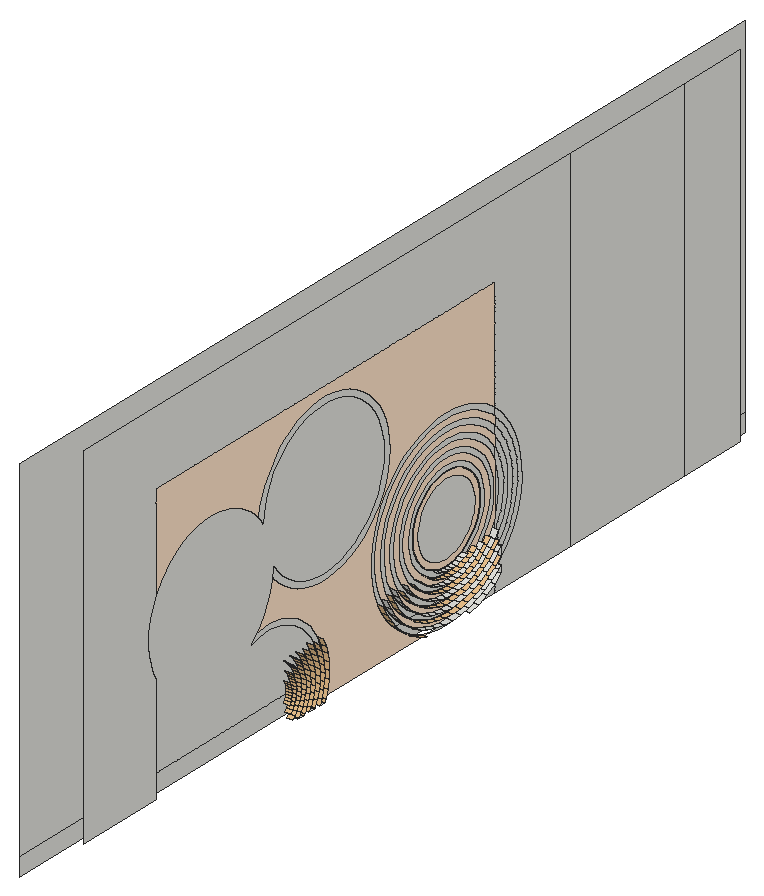
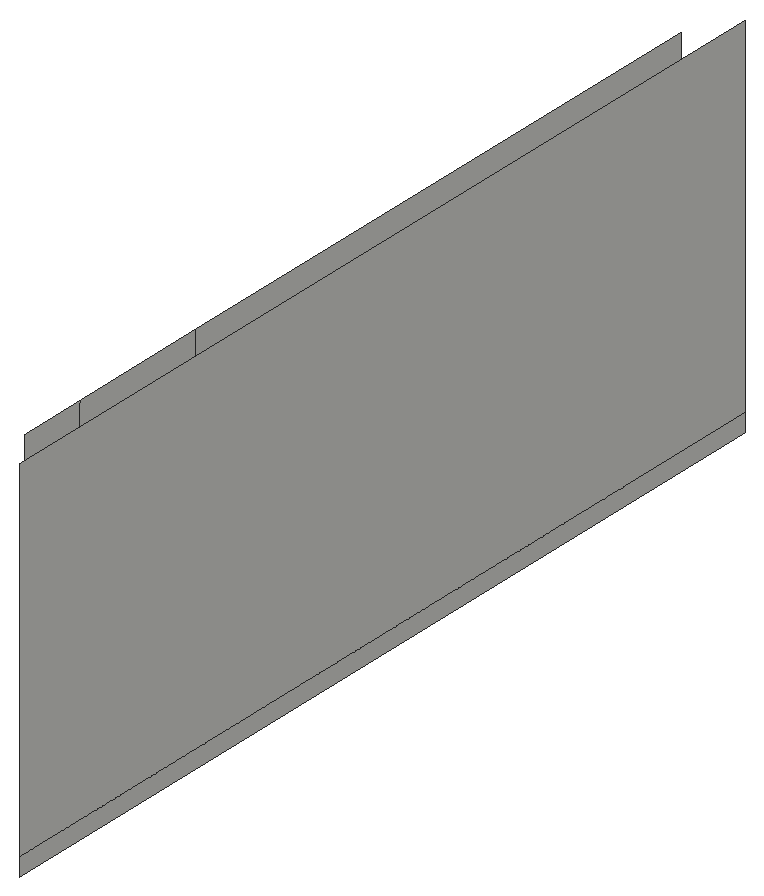
# SketchUp Ruby script. Lengths in inches.
U = 1.inch
M = Sketchup.active_model
def pt(a) = Geom::Point3d.new(a.map { |v| v * U })
def face(e, loops, mat)
  f = e.add_face(loops[0].map { |a| pt(a) })
  loops[1..].each { |l| e.add_face(l.map { |a| pt(a) }).erase! }
  f.material = f.back_material = mat if mat
  f
end
# faces: each face lists its corners as indices into pts; further lists are holes
def faces(e, pts, list, mat = nil) = list.each { |f| face(e, (f[0].is_a?(Array) ? f : [f]).map { |l| l.map { |i| pts[i] } }, mat) }
# xy, xz, yz: faces in a plane at the given z, y or x. An outline is a flat list of corners, or four numbers for a rectangle; further outlines are holes
def ring(l) = l.size == 4 ? [[l[0], l[1]], [l[2], l[1]], [l[2], l[3]], [l[0], l[3]]] : l.each_slice(2).to_a
def flat(e, list, mat, &to3) = list.each { |f| face(e, (f[0].is_a?(Array) ? f : [f]).map { |l| ring(l).map { |u, v| to3.(u, v) } }, mat) }
def xy(e, z, list, mat = nil) = flat(e, list, mat) { |x, y| [x, y, z] }
def xz(e, y, list, mat = nil) = flat(e, list, mat) { |x, z| [x, y, z] }
def yz(e, x, list, mat = nil) = flat(e, list, mat) { |y, z| [x, y, z] }
def lines(e, pts, list) = list.each { |a, b| e.add_line(pt(pts[a]), pt(pts[b])) }
# prism: a flat outline (further loops are holes) pulled along v
def prism(e, loops, v, mat = nil)
  f = face(e, loops, mat); d = Geom::Vector3d.new(v.map { |x| x * U })
  f.pushpull(f.normal.samedirection?(d) ? d.length : -d.length)
end
def box(e, o, s, mat = nil) = prism(e, [[o, [o[0] + s[0], o[1], o[2]], [o[0] + s[0], o[1] + s[1], o[2]], [o[0], o[1] + s[1], o[2]]]], [0, 0, s[2]], mat)
def at(x, y, z, deg = 0) = Geom::Transformation.translation(pt([x, y, z])) * Geom::Transformation.rotation(ORIGIN, Z_AXIS, deg.degrees)
def axes(o, x, y, z) = Geom::Transformation.new([*x, 0, *y, 0, *z, 0, *pt(o).to_a, 1])
def part(name) = M.definitions.add(name)
# library, detail: a bought-in or finely detailed component or shape, given as its bounding box
def library(name, o, s) = part(name).tap { |d| box(d.entities, o, s) }
def detail(e, o, s) = box(e.add_group.entities, o, s)
def put(e, d, t, mat = nil) = e.add_instance(d, t).tap { |i| i.material = mat if mat }
def group(e, t, mat = nil) = e.add_group.tap { |g| g.transformation = t; g.material = mat if mat }.entities
root = M.entities
M.materials.add("[Color C02]").color = [255, 228, 201]
M.materials.add("images").color = [235, 194, 141]
xy(root,0,[[183.82,104.52,185.82,107.08],[183.82,109.46,185.82,111.77],[183.82,113.98,185.82,116.09]])
xz(root,191.0625,[[183.82,6.59,185.82,9.27],[183.82,12.03,185.82,15.12]])
yz(root,174.82,[[0,-6,308.75,0],[0,0,308.75,120]])
yz(root,183.82,[[170.625,-0.85,174.39,-0.61,177.71,0,163.08,0,163.14,-0.02,166.86,-0.65],[16,0,16,120,222.875,120,222.875,0,191.0625,0,191.0625,6.59,191.43,6.86,194.16,9.47,196.57,12.37,198.62,15.54,200.29,18.92,201.5625,22.47,202.41,26.15,202.83,29.89,202.81,33.67,202.35,37.41,201.45,41.08,200.14,44.61,198.43,47.97,196.34,51.11,193.9,53.99,191.14,56.56,191.0625,56.62,191.0625,95.0625,46.5625,95.0625,46.5625,62.54,45.52,60.49,44.44,57.58,43.71,54.56,43.34,51.47,43.32,48.36,43.67,45.27,44.37,42.24,45.42,39.3125,46.5625,37.01,46.5625,0],[113.98,0,116.09,0,116.53,1.02,117.32,3.65,117.8,6.34,117.95,9.08,117.8,11.82,117.32,14.51,116.53,17.14,115.45,19.66,114.08,22.03,112.44,24.23,110.5625,26.22,108.46,27.98,106.17,29.49,103.72,30.72,101.15,31.65,98.48,32.29,95.76,32.61,93.02,32.61,90.3,32.29,90.15,32.25,89.38,31.34,87.43,29.52,88.1875,29.8,90.63,30.375,93.13,30.67,95.65,30.67,98.14,30.375,100.59,29.8,102.96,28.9375,105.2,27.81,107.3,26.43,109.23,24.81,110.96,22.98,112.46,20.96,113.71,18.79,114.71,16.48,115.43,14.07,115.87,11.59,116.01,9.08,115.87,6.57,115.43,4.09,114.71,1.68],[177.71,0,191.0625,0,191.0625,6.59,188.42,4.59,185.16,2.6875,181.71,1.17,178.1,0.07],[222.875,0,272,120],
  [272,0,295.72,120],[191.0625,6.59,191.0625,9.27,192.7,10.83,194.96,13.56,196.88,16.53,198.45,19.7,199.64,23.03,200.44,26.48,200.83,30,200.81,33.54,200.38,37.05,199.54,40.49,198.3125,43.81,196.7,46.96,194.74,49.91,192.45,52.61,191.0625,53.9,191.0625,56.62,191.14,56.56,193.9,53.99,196.34,51.11,198.43,47.97,200.14,44.61,201.45,41.08,202.35,37.41,202.81,33.67,202.83,29.89,202.41,26.15,201.5625,22.47,200.29,18.92,198.62,15.54,196.57,12.37,194.16,9.47,191.43,6.86],[191.0625,9.27,191.0625,12.03,191.23,12.2,193.34,14.74,195.15,17.52,196.61,20.48,197.72,23.59,198.47,26.82,198.83,30.1,198.8125,33.41,198.41,36.69,197.63,39.91,196.48,43.01,194.98,45.95,193.14,48.71,191.0625,51.16,191.0625,53.9,192.45,52.61,194.74,49.91,196.7,46.96,198.3125,43.81,199.54,40.49,200.38,37.05,200.81,33.54,200.83,30,200.44,26.48,199.64,23.03,198.45,19.7,196.88,16.53,194.96,13.56,192.7,10.83],[191.0625,12.03,191.0625,15.12,191.73,15.93,193.41,18.51,194.77,21.26,195.81,24.16,196.5,27.15,196.84,30.21,196.82,33.28,196.44,36.33,195.72,39.32,194.65,42.2,193.25,44.94,191.55,47.5,191.0625,48.07,191.0625,51.16,193.14,48.71,194.98,45.95,196.48,43.01,197.63,39.91,198.41,36.69,198.8125,33.41,198.83,30.1,198.47,26.82,197.72,23.59,196.61,20.48,195.15,17.52,193.34,14.74,191.23,12.2],[191.0625,15.12,191.0625,18.5625,191.67,19.5,192.93,22.04,193.89,24.72,194.53,27.49,194.84,30.3125,194.82,33.15,194.48,35.97,193.8,38.74,192.82,41.4,191.53,43.93,191.0625,44.63,191.0625,48.07,191.55,47.5,193.25,44.94,194.65,42.2,195.72,39.32,196.44,36.33,196.82,33.28,196.84,30.21,196.5,27.15,195.81,24.16,194.77,21.26,193.41,18.51,191.73,15.93],
  [[170.52,17.15,172.19,17.26,173.85,17.5625,175.45,18.05,176.99,18.73,178.4375,19.57,179.78,20.58,180.99,21.74,182.07,23.04,182.98,24.44,183.72,25.95,184.29,27.53,184.67,29.17,184.85,30.83,184.84,32.51,184.64,34.18,184.24,35.8125,183.66,37.39,182.89,38.88,181.96,40.28,180.88,41.56,179.65,42.7,178.3,43.7,176.84,44.53,175.29,45.18,173.68,45.66,172.03,45.9375,170.35,46.03,168.67,45.92,167.02,45.62,165.42,45.125,163.88,44.45,162.43,43.6,161.09,42.59,159.875,41.43,158.8,40.14,157.89,38.73,157.14,37.23,156.58,35.65,156.2,34.01,156.02,32.34,156.03,30.66,156.23,29,156.63,27.37,157.21,25.79,157.97,24.3,158.9,22.9,159.99,21.62,161.22,20.47,162.57,19.48,164.03,18.65,165.58,17.99,167.1875,17.52,168.84,17.24],[170.52,17.16,168.84,17.24,167.1875,17.52,165.58,18,164.03,18.65,162.57,19.48,161.22,20.48,159.99,21.62,158.91,22.9,157.98,24.3,157.21,25.79,156.63,27.37,156.23,29,156.03,30.66,156.02,32.34,156.2,34.01,156.58,35.65,157.15,37.23,157.89,38.73,158.81,40.14,159.875,41.43,161.09,42.59,162.43,43.6,163.88,44.45,165.42,45.125,167.02,45.61,168.67,45.92,170.35,46.02,172.03,45.94,173.68,45.65,175.29,45.18,176.84,44.53,178.29,43.7,179.65,42.7,180.875,41.56,181.96,40.28,182.89,38.88,183.65,37.38,184.24,35.8125,184.63,34.18,184.84,32.51,184.85,30.84,184.66,29.17,184.29,27.53,183.72,25.95,182.98,24.45,182.0625,23.04,180.99,21.75,179.78,20.59,178.4375,19.58,176.99,18.73,175.45,18.05,173.85,17.5625,172.19,17.26]],[191.0625,18.5625,191.0625,22.77,191.09,22.82,191.97,25.28,192.55,27.82,192.84,30.42,192.83,33.03,192.51,35.62,191.89,38.15,191.0625,40.39,191.0625,44.63,191.53,43.93,192.82,41.4,193.8,38.74,194.48,35.97,194.82,33.15,194.84,30.3125,194.53,27.49,193.89,24.72,192.93,22.04,191.67,19.5],[191.0625,22.77,191.0625,40.39,191.89,38.15,192.51,35.62,192.83,33.03,192.84,30.42,192.55,27.82,191.97,25.28,191.09,22.82],[116.6,35.71,119.85,35.71,123.08,36.08,126.24,36.82,129.3,37.93,132.2,39.38,134.92,41.16,137.41,43.25,139.64,45.61,141.59,48.21,143.21,51.02,144.51,54,145.44,57.11,146.01,60.31,146.2,63.55,146.02,66.8,145.46,70,144.53,73.11,143.25,76.09,141.63,78.91,139.7,81.52,137.47,83.88,134.99,85.98,132.27,87.77,129.375,89.23,126.32,90.34,123.16,91.1,119.9375,91.48,116.6875,91.48,113.46,91.11,110.3,90.37,107.24,89.26,104.34,87.81,101.62,86.03,99.13,83.94,96.9,81.58,94.95,78.98,93.33,76.17,92.04,73.1875,91.1,70.08,90.53,66.88,90.53,66.87,91.55,65.64,92.38,64.36,92.52,66.64,93.04,69.61,93.91,72.5,95.11,75.27,96.625,77.88,98.43,80.29,100.5,82.49,102.81,84.42,105.34,86.07,108.03,87.42,110.87,88.45,113.81,89.14,116.8,89.49,119.82,89.48,122.8125,89.13,125.75,88.43,128.58,87.39,131.27,86.03,133.79,84.375,136.1,82.43,138.16,80.23,139.96,77.8125,141.46,75.2,142.65,72.43,143.51,69.54,144.03,66.57,144.2,63.56,144.02,60.55,143.5,57.58,142.63,54.6875,141.43,51.92,139.92,49.3125,138.11,46.89,136.04,44.7,133.73,42.77,131.2,41.12,128.51,39.77,125.67,38.74,122.74,38.05,119.74,37.7,116.72,37.71,113.73,38.0625,110.8,38.76,107.96,39.8,105.27,41.15,102.75,42.82,100.45,44.76,98.38,46.95,96.71,49.2,96.71,48.1,96.47,46.17,96.84,45.67,99.07,43.3,101.56,41.21,104.27,39.42,107.17,37.96,110.22,36.85,113.38,36.09]])
yz(root,183.82,[[116.09,0,163.08,0,159.52,1.04,156.05,2.52,152.77,4.38,149.73,6.62,146.97,9.19,144.53,12.07,142.4375,15.2,140.73,18.57,139.41,22.1,138.52,25.77,138.0625,29.51,138.04,33.28,138.46,37.03,139.31,40.71,140.57,44.26,142.25,47.64,144.3,50.81,146.71,53.71,149.4375,56.3125,152.45,58.58,155.71,60.49,159.16,62,162.77,63.11,166.48,63.78,170.24,64.03,174.01,63.83,177.73,63.2,181.35,62.14,184.82,60.66,188.1,58.8,191.0625,56.62,191.0625,95.0625,46.5625,95.0625,46.5625,62.54,46.93,63.27,48.65,65.86,50.66,68.23,52.94,70.35,55.4375,72.19,58.14,73.74,61,74.95,63.98,75.83,67.05,76.36,70.15,76.52,73.26,76.32,76.32,75.77,79.29,74.86,82.14,73.62,84.82,72.05,87.31,70.18,89.56,68.04,90.53,66.87,90.53,66.88,91.1,70.08,92.04,73.1875,93.33,76.17,94.95,78.98,96.9,81.58,99.13,83.94,101.62,86.03,104.34,87.81,107.24,89.26,110.3,90.37,113.46,91.11,116.6875,91.48,119.9375,91.48,123.16,91.1,126.32,90.34,129.375,89.23,132.27,87.77,134.99,85.98,137.47,83.88,139.7,81.52,141.63,78.91,143.25,76.09,144.53,73.11,145.46,70,146.02,66.8,146.2,63.55,146.01,60.31,145.44,57.11,144.51,54,143.21,51.02,141.59,48.21,139.64,45.61,137.41,43.25,134.92,41.16,132.2,39.38,129.3,37.93,126.24,36.82,123.08,36.08,119.85,35.71,116.6,35.71,113.38,36.09,110.22,36.85,107.17,37.96,104.27,39.42,101.56,41.21,99.07,43.3,96.84,45.67,96.47,46.17,96.33,45.01,95.6,41.99,94.52,39.07,93.11,36.3,91.39,33.71,90.15,32.25,90.3,32.29,93.02,32.61,95.76,32.61,98.48,32.29,101.15,31.65,103.72,30.72,106.17,29.49,108.46,27.98,110.5625,26.22,112.44,24.23,114.08,22.03,115.45,19.66,116.53,17.14,117.32,14.51,117.8,11.82,117.95,9.08,117.8,6.34,117.32,3.65,116.53,1.02],[170.61,1.15,174.15,1.38,177.63,2.01,181.01,3.05,184.25,4.47,187.31,6.26,190.14,8.39,191.0625,9.27,191.0625,12.03,188.84,9.91,186.2,7.92,183.35,6.25,180.32,4.92,177.16,3.96,173.9,3.36,170.6,3.15,167.3,3.33,164.04,3.88,160.87,4.81,157.82,6.1,154.95,7.74,152.28,9.7,149.87,11.95,147.72,14.47,145.89,17.23,144.39,20.17,143.24,23.27,142.46,26.49,142.06,29.77,142.04,33.08,142.4,36.36,143.14,39.58,144.26,42.7,145.72,45.66,147.52,48.4375,149.63,50.98,152.03,53.27,154.67,55.26,157.52,56.93,160.55,58.25,163.71,59.22,166.97,59.8125,170.27,60.03,173.57,59.85,176.83,59.3,180,58.37,183.05,57.08,185.92,55.44,188.58,53.48,191,51.23,191.0625,51.16,191.0625,53.9,189.86,55.02,187.01,57.12,183.93,58.87,180.68,60.25,177.28,61.25,173.79,61.84,170.25,62.03,166.72,61.8,163.24,61.16,159.86,60.13,156.61,58.71,153.56,56.92,150.73,54.79,148.17,52.35,145.91,49.62,143.99,46.65,142.42,43.48,141.22,40.15,140.43,36.7,140.04,33.18,140.06,29.64,140.49,26.125,141.33,22.6875,142.56,19.37,144.16,16.22,146.13,13.27,148.42,10.57,151.01,8.16,153.86,6.0625,156.93,4.31,160.19,2.93,163.59,1.93,167.08,1.34],[170.59,5.15,173.66,5.35,176.68,5.9,179.62,6.8,182.4375,8.03,185.09,9.59,187.55,11.4375,189.77,13.5625,191.0625,15.12,191.0625,18.5625,190.12,17.11,188.31,14.92,186.25,12.96,183.98,11.25,181.53,9.82,178.93,8.68,176.21,7.84,173.41,7.33,170.58,7.15,167.74,7.3,164.9375,7.78,162.21,8.58,159.6,9.6875,157.125,11.09,154.84,12.78,152.76,14.71,150.92,16.88,149.34,19.25,148.05,21.78,147.07,24.44,146.39,27.2,146.05,30.02,146.03,32.87,146.34,35.69,146.98,38.46,147.9375,41.14,149.2,43.68,150.75,46.07,152.56,48.25,154.62,50.22,156.89,51.93,159.34,53.36,161.94,54.5,164.66,55.33,167.45,55.84,170.29,56.03,173.13,55.88,175.93,55.4,178.66,54.6,181.27,53.49,183.74,52.09,186.03,50.4,188.11,48.46,189.95,46.3,191.0625,44.63,191.0625,48.07,189.56,49.84,187.31,51.94,184.83,53.76,182.16,55.28,179.33,56.49,176.38,57.35,173.35,57.87,170.28,58.03,167.21,57.83,164.1875,57.28,161.25,56.38,158.43,55.14,155.78,53.59,153.32,51.74,151.1,49.62,149.14,47.25,147.46,44.67,146.1,41.92,145.0625,39.02,144.37,36.03,144.03,32.97,144.05,29.9,144.43,26.84,145.15,23.86,146.22,20.97,147.62,18.24,149.32,15.68,151.3125,13.33,153.56,11.24,156.04,9.42,158.71,7.89,161.54,6.69,164.49,5.83,167.52,5.3125],[[170.57,9.15,173.17,9.32,175.74,9.79,178.23,10.55,180.62,11.6,182.875,12.92,184.96,14.49,186.85,16.29,188.51,18.3,189.93,20.49,191.0625,22.77,191.0625,40.39,190.98,40.6,189.8,42.92,188.35,45.09,186.66,47.08,184.76,48.86,182.65,50.41,180.39,51.7,177.98,52.72,175.48,53.45,172.91,53.89,170.3,54.03,167.7,53.86,165.13,53.39,162.64,52.63,160.25,51.58,157.99,50.26,155.91,48.69,154.02,46.89,152.36,44.88,150.9375,42.69,149.78,40.35,148.9,37.9,148.32,35.35,148.03,32.76,148.04,30.15,148.36,27.5625,148.98,25.03,149.88,22.58,151.07,20.26,152.52,18.08,154.2,16.1,156.11,14.32,158.22,12.77,160.48,11.48,162.88,10.46,165.39,9.73,167.96,9.29],[170.55,11.15,168.18,11.28,165.84,11.68,163.56,12.34,161.37,13.27,159.3,14.45,157.39,15.86,155.65,17.48,154.11,19.29,152.8,21.27,151.72,23.38,150.89,25.61,150.33,27.92,150.04,30.28,150.02,32.66,150.29,35.02,150.82,37.34,151.62,39.57,152.67,41.7,153.97,43.7,155.49,45.53,157.21,47.17,159.1,48.6,161.15,49.8,163.33,50.75,165.6,51.45,167.94,51.875,170.3125,52.03,172.6875,51.9,175.03,51.5,177.3125,50.84,179.5,49.91,181.5625,48.73,183.48,47.32,185.22,45.7,186.76,43.89,188.07,41.91,189.15,39.79,189.98,37.57,190.54,35.26,190.83,32.9,190.84,30.52,190.58,28.16,190.05,25.84,189.25,23.61,188.19,21.48,186.9,19.48,185.38,17.65,183.66,16.01,181.77,14.58,179.71,13.38,177.54,12.43,175.26,11.73,172.93,11.3]],[[170.54,13.15,172.68,13.29,174.79,13.67,176.84,14.3,178.81,15.16,180.66,16.25,182.37,17.54,183.92,19.02,185.29,20.67,186.46,22.46,187.41,24.39,188.13,26.41,188.61,28.49,188.85,30.625,188.83,32.77,188.57,34.9,188.07,36.98,187.32,38.99,186.35,40.9,185.16,42.6875,183.77,44.32,182.2,45.78,180.47,47.05,178.61,48.11,176.64,48.95,174.58,49.55,172.47,49.91,170.33,50.03,168.1875,49.89,166.08,49.5,164.03,48.88,162.0625,48.02,160.21,46.93,158.5,45.64,156.95,44.16,155.58,42.51,154.41,40.71,153.46,38.79,152.74,36.77,152.26,34.68,152.02,32.55,152.03,30.41,152.3,28.28,152.8,26.2,153.55,24.1875,154.52,22.28,155.71,20.49,157.1,18.86,158.67,17.4,160.39,16.125,162.26,15.0625,164.23,14.23,166.29,13.625,168.4,13.26],[170.53,15.15,168.62,15.25,166.74,15.57,164.9,16.11,163.14,16.86,161.48,17.8,159.94,18.94,158.54,20.24,157.31,21.7,156.25,23.29,155.38,24.99,154.72,26.78,154.26,28.64,154.03,30.54,154.02,32.45,154.23,34.35,154.66,36.21,155.3,38.01,156.15,39.72,157.19,41.33,158.41,42.8,159.79,44.12,161.32,45.27,162.97,46.23,164.72,47,166.55,47.5625,168.43,47.9,170.34,48.03,172.25,47.93,174.13,47.61,175.96,47.07,177.72,46.32,179.39,45.375,180.93,44.24,182.32,42.94,183.5625,41.48,184.62,39.89,185.49,38.1875,186.15,36.4,186.6,34.54,186.84,32.64,186.85,30.73,186.64,28.83,186.21,26.97,185.57,25.17,184.72,23.45,183.68,21.85,182.46,20.38,181.07,19.06,179.55,17.91,177.9,16.94,176.15,16.18,174.32,15.62,172.4375,15.27]],
  [[170.52,17.16,172.19,17.26,173.85,17.5625,175.45,18.05,176.99,18.73,178.4375,19.58,179.78,20.59,180.99,21.75,182.0625,23.04,182.98,24.45,183.72,25.95,184.29,27.53,184.66,29.17,184.85,30.84,184.84,32.51,184.63,34.18,184.24,35.8125,183.65,37.38,182.89,38.88,181.96,40.28,180.875,41.56,179.65,42.7,178.29,43.7,176.84,44.53,175.29,45.18,173.68,45.65,172.03,45.94,170.35,46.02,168.67,45.92,167.02,45.61,165.42,45.125,163.88,44.45,162.43,43.6,161.09,42.59,159.875,41.43,158.81,40.14,157.89,38.73,157.15,37.23,156.58,35.65,156.2,34.01,156.02,32.34,156.03,30.66,156.23,29,156.63,27.37,157.21,25.79,157.98,24.3,158.91,22.9,159.99,21.62,161.22,20.48,162.57,19.48,164.03,18.65,165.58,18,167.1875,17.52,168.84,17.24],[170.51,19.15,169.0625,19.23,167.64,19.47,166.25,19.875,164.92,20.44,163.66,21.16,162.5,22.01,161.4375,23,160.5,24.1,159.7,25.31,159.04,26.6,158.54,27.95,158.2,29.36,158.02,30.79,158.01,32.24,158.17,33.68,158.5,35.09,158.99,36.45,159.625,37.74,160.41,38.96,161.34,40.07,162.38,41.07,163.54,41.94,164.79,42.67,166.11,43.25,167.49,43.67,168.92,43.93,170.36,44.03,171.81,43.95,173.23,43.71,174.62,43.3,175.95,42.74,177.21,42.02,178.37,41.16,179.43,40.18,180.37,39.08,181.17,37.87,181.83,36.58,182.33,35.23,182.67,33.82,182.85,32.39,182.85,30.9375,182.7,29.5,182.37,28.09,181.88,26.73,181.24,25.43,180.45,24.22,179.53,23.11,178.49,22.11,177.33,21.24,176.08,20.51,174.76,19.93,173.375,19.5,171.95,19.24]]],"[Color C02]")
p = [[183.82,104.83,0.32],[183.82,104.52,0],[185.82,104.52,0],[185.82,104.83,0.32],[183.82,107.08,0],[183.82,107.44,0.49],
  [185.82,107.44,0.49],[185.82,107.08,0],[183.82,110.14,1.17],[183.82,109.46,0],[185.82,109.46,0],[185.82,110.14,1.17],
  [183.82,111.77,0],[183.82,111.93,0.27],[185.82,111.93,0.27],[185.82,111.77,0],[183.82,114.71,1.68],[183.82,113.98,0],
  [185.82,113.98,0],[185.82,114.71,1.68],[183.82,116.09,0],[183.82,116.53,1.02],[185.82,116.53,1.02],[185.82,116.09,0],
  [183.82,178.1,0.07],[183.82,181.71,1.17],[185.82,181.71,1.17],[185.82,178.1,0.07],[183.82,105.77,1.59],[185.82,105.77,1.59],
  [183.82,112.83,2.37],[185.82,112.83,2.37],[183.82,108.35,2.07],[185.82,108.35,2.07],[183.82,102.37,0.625],[183.82,103.3,1.61],
  [185.82,103.3,1.61],[185.82,102.37,0.625],[183.82,117.32,3.65],[185.82,117.32,3.65],[183.82,156.05,2.52],[183.82,159.52,1.04],
  [185.82,159.52,1.04],[185.82,156.05,2.52],[183.82,110.95,3.05],[185.82,110.95,3.05],[183.82,170.61,1.15],[183.82,167.08,1.34],
  [185.82,167.08,1.34],[185.82,170.61,1.15],[183.82,174.15,1.38],[185.82,174.15,1.38],[183.82,185.16,2.6875],[185.82,185.16,2.6875],
  [183.82,163.59,1.93],[185.82,163.59,1.93],[183.82,177.63,2.01],[185.82,177.63,2.01],[183.82,104.1,2.69],[185.82,104.1,2.69],
  [183.82,106.57,2.97],[185.82,106.57,2.97],[183.82,115.43,4.09],[185.82,115.43,4.09],[183.82,160.19,2.93],[185.82,160.19,2.93],
  [183.82,181.01,3.05],[185.82,181.01,3.05],[183.82,109.07,3.74],[185.82,109.07,3.74],[183.82,113.49,4.55],[185.82,113.49,4.55],
  [183.82,152.77,4.38],[185.82,152.77,4.38],[183.82,104.78,3.86],[185.82,104.78,3.86],[183.82,188.42,4.59],[185.82,188.42,4.59],
  [183.82,102.43,3.79],[183.82,101.76,2.89],[185.82,101.76,2.89],[185.82,102.43,3.79],[183.82,156.93,4.31],[185.82,156.93,4.31],
  [183.82,107.19,4.42],[185.82,107.19,4.42],[183.82,184.25,4.47],[185.82,184.25,4.47],[183.82,111.54,5.02],[185.82,111.54,5.02],
  [183.82,167.3,3.33],[183.82,170.6,3.15],[185.82,170.6,3.15],[185.82,167.3,3.33],[183.82,173.9,3.36],[185.82,173.9,3.36],
  [183.82,164.04,3.88],[185.82,164.04,3.88],[183.82,177.16,3.96],[185.82,177.16,3.96],[183.82,117.8,6.34],[185.82,117.8,6.34],
  [183.82,109.59,5.48],[185.82,109.59,5.48],[183.82,102.99,4.76],[185.82,102.99,4.76],[183.82,105.3125,5.1],[185.82,105.3125,5.1],
  [183.82,160.87,4.81],[185.82,160.87,4.81],[183.82,180.32,4.92],[185.82,180.32,4.92],[183.82,115.87,6.57],[185.82,115.87,6.57],
  [183.82,153.86,6.0625],[185.82,153.86,6.0625],[183.82,107.65,5.9375],[185.82,107.65,5.9375],[183.82,149.73,6.62],[185.82,149.73,6.62],
  [183.82,187.31,6.26],[185.82,187.31,6.26],[183.82,113.88,6.8],[185.82,113.88,6.8],[183.82,191.0625,6.59],[185.82,191.0625,6.59],
  [183.82,103.43,5.79],[185.82,103.43,5.79],[183.82,157.82,6.1],[185.82,157.82,6.1],[183.82,183.35,6.25],[185.82,183.35,6.25],
  [183.82,111.9,7.03],[185.82,111.9,7.03],[183.82,105.7,6.4],[185.82,105.7,6.4],[183.82,170.59,5.15],[183.82,167.52,5.3125],
  [185.82,167.52,5.3125],[185.82,170.59,5.15],[183.82,173.66,5.35],[185.82,173.66,5.35],[183.82,164.49,5.83],[185.82,164.49,5.83],
  [183.82,176.68,5.9],[185.82,176.68,5.9],[183.82,109.91,7.27],[185.82,109.91,7.27],[183.82,101.2,5.66],[183.82,101.55,6.47],
  [185.82,101.55,6.47],[185.82,101.2,5.66],[183.82,103.76,6.86],[185.82,103.76,6.86],[183.82,161.54,6.69],[185.82,161.54,6.69],
  [183.82,107.92,7.5],[185.82,107.92,7.5],[183.82,179.62,6.8],[185.82,179.62,6.8],[183.82,151.01,8.16],[185.82,151.01,8.16],
  [183.82,154.95,7.74],[185.82,154.95,7.74],[183.82,117.95,9.08],[185.82,117.95,9.08],[183.82,186.2,7.92],[185.82,186.2,7.92],
  [183.82,190.14,8.39],[185.82,190.14,8.39],[183.82,105.9375,7.73],[185.82,105.9375,7.73],[183.82,101.81,7.32],[185.82,101.81,7.32],
  [183.82,116.01,9.08],[185.82,116.01,9.08],[183.82,146.97,9.19],[185.82,146.97,9.19],[183.82,158.71,7.89],[185.82,158.71,7.89],
  [183.82,114.01,9.08],[185.82,114.01,9.08],[183.82,182.4375,8.03],[185.82,182.4375,8.03],[183.82,103.95,7.96],[185.82,103.95,7.96],
  [183.82,112.01,9.08],[185.82,112.01,9.08],[183.82,167.74,7.3],[183.82,170.58,7.15],[185.82,170.58,7.15],[185.82,167.74,7.3],
  [183.82,173.41,7.33],[185.82,173.41,7.33],[183.82,101.96,8.19],[185.82,101.96,8.19],[183.82,110.01,9.08],[185.82,110.01,9.08],
  [183.82,164.9375,7.78],[185.82,164.9375,7.78],[183.82,176.21,7.84],[185.82,176.21,7.84],[183.82,108.01,9.08],[185.82,108.01,9.08],
  [183.82,106.01,9.08],[185.82,106.01,9.08],[183.82,152.28,9.7],[185.82,152.28,9.7],[183.82,162.21,8.58],[185.82,162.21,8.58],
  [183.82,178.93,8.68],[185.82,178.93,8.68],[183.82,156.04,9.42],[185.82,156.04,9.42],[183.82,188.84,9.91],[185.82,188.84,9.91],
  [183.82,104.01,9.08],[185.82,104.01,9.08],[183.82,185.09,9.59],[185.82,185.09,9.59],[183.82,102.01,9.08],[185.82,102.01,9.08],
  [183.82,148.42,10.57],[185.82,148.42,10.57],[183.82,191.0625,9.27],[185.82,191.0625,9.27],[183.82,159.6,9.6875],[185.82,159.6,9.6875],
  [183.82,181.53,9.82],[185.82,181.53,9.82],[183.82,101.96,9.97],[185.82,101.96,9.97],[183.82,103.95,10.2],[185.82,103.95,10.2],
  [183.82,105.9375,10.43],[185.82,105.9375,10.43],[183.82,107.92,10.66],[185.82,107.92,10.66],[183.82,109.91,10.89],[185.82,109.91,10.89],
  [183.82,111.9,11.125],[185.82,111.9,11.125],[183.82,113.88,11.36],[185.82,113.88,11.36],[183.82,115.87,11.59],[185.82,115.87,11.59],
  [183.82,117.8,11.82],[185.82,117.8,11.82],[183.82,144.53,12.07],[185.82,144.53,12.07],[183.82,170.57,9.15],[183.82,167.96,9.29],
  [185.82,167.96,9.29],[185.82,170.57,9.15],[183.82,173.17,9.32],[185.82,173.17,9.32],[183.82,165.39,9.73],[185.82,165.39,9.73],
  [183.82,175.74,9.79],[185.82,175.74,9.79],[183.82,153.56,11.24],[185.82,153.56,11.24],[183.82,187.55,11.4375],[185.82,187.55,11.4375],
  [183.82,149.87,11.95],[185.82,149.87,11.95],[183.82,157.125,11.09],[185.82,157.125,11.09],[183.82,162.88,10.46],[185.82,162.88,10.46],
  [183.82,178.23,10.55],[185.82,178.23,10.55],[183.82,183.98,11.25],[185.82,183.98,11.25],[183.82,191.0625,12.03],[185.82,191.0625,12.03],
  [183.82,101.81,10.84],[185.82,101.81,10.84],[183.82,103.76,11.3],[185.82,103.76,11.3],[183.82,105.7,11.76],[185.82,105.7,11.76],
  [183.82,160.48,11.48],[185.82,160.48,11.48],[183.82,146.13,13.27],[185.82,146.13,13.27],[183.82,180.62,11.6],[185.82,180.62,11.6],
  [183.82,107.65,12.22],[185.82,107.65,12.22],[183.82,101.55,11.6875],[185.82,101.55,11.6875],[183.82,109.59,12.68],[185.82,109.59,12.68],
  [183.82,111.54,13.14],[185.82,111.54,13.14],[183.82,154.84,12.78],[185.82,154.84,12.78],[183.82,151.3125,13.33],[185.82,151.3125,13.33],
  [183.82,168.18,11.28],[183.82,170.55,11.15],[185.82,170.55,11.15],[185.82,168.18,11.28],[183.82,172.93,11.3],[185.82,172.93,11.3],
  [183.82,103.43,12.37],[185.82,103.43,12.37],[183.82,165.84,11.68],[185.82,165.84,11.68],[183.82,175.26,11.73],[185.82,175.26,11.73],
  [183.82,186.25,12.96],[185.82,186.25,12.96],[183.82,113.49,13.61],[185.82,113.49,13.61],[183.82,189.77,13.5625],[185.82,189.77,13.5625],
  [183.82,158.22,12.77],[185.82,158.22,12.77],[183.82,115.43,14.07],[185.82,115.43,14.07],[183.82,182.875,12.92],[185.82,182.875,12.92],
  [183.82,101.2,12.5],[185.82,101.2,12.5],[183.82,163.56,12.34],[185.82,163.56,12.34],[183.82,177.54,12.43],[185.82,177.54,12.43],
  [183.82,105.3125,13.06],[185.82,105.3125,13.06],[183.82,117.32,14.51],[185.82,117.32,14.51],[183.82,147.72,14.47],[185.82,147.72,14.47],
  [183.82,142.4375,15.2],[185.82,142.4375,15.2],[183.82,107.19,13.74],[185.82,107.19,13.74],[183.82,161.37,13.27],[185.82,161.37,13.27],
  [183.82,102.99,13.4],[185.82,102.99,13.4],[183.82,179.71,13.38],[185.82,179.71,13.38],[183.82,109.07,14.42],[185.82,109.07,14.42],
  [183.82,152.76,14.71],[185.82,152.76,14.71],[183.82,156.11,14.32],[185.82,156.11,14.32],[183.82,184.96,14.49],[185.82,184.96,14.49],
  [183.82,188.31,14.92],[185.82,188.31,14.92],[183.82,104.78,14.3],[185.82,104.78,14.3],[183.82,110.95,15.11],[185.82,110.95,15.11],
  [183.82,170.54,13.15],[183.82,168.4,13.26],[185.82,168.4,13.26],[185.82,170.54,13.15],[183.82,172.68,13.29],[185.82,172.68,13.29],
  [183.82,144.16,16.22],[185.82,144.16,16.22],[183.82,149.32,15.68],[185.82,149.32,15.68],[183.82,159.3,14.45],[185.82,159.3,14.45],
  [183.82,166.29,13.625],[185.82,166.29,13.625],[183.82,174.79,13.67],[185.82,174.79,13.67],[183.82,102.43,14.37],[185.82,102.43,14.37],
  [183.82,181.77,14.58],[185.82,181.77,14.58],[183.82,112.83,15.79],[185.82,112.83,15.79],[183.82,164.23,14.23],[185.82,164.23,14.23],
  [183.82,191.0625,15.12],[185.82,191.0625,15.12],[183.82,106.57,15.19],[185.82,106.57,15.19],[183.82,176.84,14.3],[185.82,176.84,14.3],
  [183.82,114.71,16.48],[185.82,114.71,16.48],[183.82,162.26,15.0625],[185.82,162.26,15.0625],[183.82,104.1,15.47],[185.82,104.1,15.47],
  [183.82,154.2,16.1],[185.82,154.2,16.1],[183.82,178.81,15.16],[185.82,178.81,15.16],[183.82,101.76,15.27],[185.82,101.76,15.27],
  [183.82,108.35,16.09],[185.82,108.35,16.09],[183.82,157.39,15.86],[185.82,157.39,15.86],[183.82,116.53,17.14],[185.82,116.53,17.14],
  [183.82,145.89,17.23],[185.82,145.89,17.23],[183.82,186.85,16.29],[185.82,186.85,16.29],[183.82,183.66,16.01],[185.82,183.66,16.01],
  [183.82,150.92,16.88],[185.82,150.92,16.88],[183.82,190.12,17.11],[185.82,190.12,17.11],[183.82,110.14,16.99],[185.82,110.14,16.99],
  [183.82,160.39,16.125],[185.82,160.39,16.125],[183.82,105.77,16.57],[185.82,105.77,16.57],[183.82,140.73,18.57],[185.82,140.73,18.57],
  [183.82,168.62,15.25],[183.82,170.53,15.15],[185.82,170.53,15.15],[185.82,168.62,15.25],[183.82,172.4375,15.27],[185.82,172.4375,15.27],
  [183.82,180.66,16.25],[185.82,180.66,16.25],[183.82,166.74,15.57],[185.82,166.74,15.57],[183.82,174.32,15.62],[185.82,174.32,15.62],
  [183.82,103.3,16.55],[185.82,103.3,16.55],[183.82,164.9,16.11],[185.82,164.9,16.11],[183.82,176.15,16.18],[185.82,176.15,16.18],
  [183.82,147.62,18.24],[185.82,147.62,18.24],[183.82,111.93,17.89],[185.82,111.93,17.89],[183.82,155.65,17.48],[185.82,155.65,17.48],
  [183.82,185.38,17.65],[185.82,185.38,17.65],[183.82,107.44,17.67],[185.82,107.44,17.67],[183.82,152.52,18.08],[185.82,152.52,18.08],
  [183.82,158.67,17.4],[185.82,158.67,17.4],[183.82,163.14,16.86],[185.82,163.14,16.86],[183.82,142.56,19.37],[185.82,142.56,19.37],
  [183.82,177.9,16.94],[185.82,177.9,16.94],[183.82,182.37,17.54],[185.82,182.37,17.54],[183.82,188.51,18.3],[185.82,188.51,18.3],
  [183.82,113.71,18.79],[185.82,113.71,18.79],[183.82,102.37,17.54],[185.82,102.37,17.54],[183.82,104.83,17.84],[185.82,104.83,17.84],
  [183.82,149.34,19.25],[185.82,149.34,19.25],[183.82,161.48,17.8],[185.82,161.48,17.8],[183.82,179.55,17.91],[185.82,179.55,17.91],
  [183.82,109.12,18.77],[185.82,109.12,18.77],[183.82,115.45,19.66],[185.82,115.45,19.66],[183.82,144.39,20.17],[185.82,144.39,20.17],
  [183.82,168.84,17.24],[183.82,167.1875,17.52],[185.82,167.1875,17.52],[185.82,168.84,17.24],[183.82,170.52,17.15],[185.82,170.52,17.15],
  [183.82,172.19,17.26],[185.82,172.19,17.26],[183.82,173.85,17.5625],[185.82,173.85,17.5625],[183.82,157.1,18.86],[185.82,157.1,18.86],
  [183.82,101.33,18.4],[185.82,101.33,18.4],[183.82,154.11,19.29],[185.82,154.11,19.29],[183.82,165.58,17.99],[185.82,165.58,17.99],
  [183.82,183.92,19.02],[185.82,183.92,19.02],[183.82,175.45,18.05],[185.82,175.45,18.05],[183.82,106.36,19.125],[185.82,106.36,19.125],
  [183.82,186.9,19.48],[185.82,186.9,19.48],[183.82,103.74,18.99],[185.82,103.74,18.99],[183.82,159.94,18.94],[185.82,159.94,18.94],
  [183.82,110.79,19.86],[185.82,110.79,19.86],[183.82,181.07,19.06],[185.82,181.07,19.06],[183.82,164.03,18.65],[185.82,164.03,18.65],
  [183.82,151.07,20.26],[185.82,151.07,20.26],[183.82,176.99,18.73],[185.82,176.99,18.73],[183.82,146.22,20.97],[185.82,146.22,20.97],
  [183.82,189.93,20.49],[185.82,189.93,20.49]]
faces(root,p,[[0,1,2,3],[4,5,6,7],[8,9,10,11],[12,13,14,15],[16,17,18,19],[20,21,22,23],[28,0,3,29],[13,30,31,14],
  [5,32,33,6],[34,35,36,37],[21,38,39,22],[40,41,42,43],[44,8,11,45],[35,58,59,36],[60,28,29,61],[62,16,19,63],
  [32,68,69,33],[30,70,71,31],[72,40,43,73],[58,74,75,59],[78,79,80,81],[84,60,61,85],[88,44,45,89],[90,91,92,93],
  [91,94,95,92],[96,90,93,97],[94,98,99,95],[38,100,101,39],[68,102,103,69],[104,78,81,105],[74,106,107,75],[108,96,97,109],
  [98,110,111,99],[112,62,63,113],[116,84,85,117],[118,72,73,119],[70,122,123,71],[126,104,105,127],[128,108,109,129],[110,130,131,111],
  [132,88,89,133],[106,134,135,107],[102,146,147,103],[148,149,150,151],[152,126,127,153],[156,116,117,157],[162,128,129,163],[100,164,165,101],
  [130,166,167,131],[134,170,171,135],[149,172,173,150],[174,112,113,175],[176,118,119,177],[122,180,181,123],[184,152,153,185],[186,132,133,187],
  [188,189,190,191],[189,192,193,190],[172,194,195,173],[146,196,197,147],[198,188,191,199],[192,200,201,193],[202,156,157,203],[170,204,205,171],
  [206,162,163,207],[208,198,199,209],[200,210,211,201],[166,214,215,167],[216,184,185,217],[194,220,221,195],[226,208,209,227],[210,228,229,211],
  [220,230,231,221],[232,216,217,233],[204,234,235,205],[236,202,203,237],[196,238,239,197],[240,186,187,241],[180,242,243,181],[244,174,175,245],
  [164,246,247,165],[248,176,177,249],[264,206,207,265],[266,226,227,267],[228,272,273,229],[214,274,275,215],[230,276,277,231],[278,232,233,279],
  [234,280,281,235],[288,236,237,289],[276,290,291,277],[238,292,293,239],[294,240,241,295],[296,266,267,297],[300,301,302,303],[301,304,305,302],
  [306,278,279,307],[308,300,303,309],[304,310,311,305],[272,312,313,273],[242,314,315,243],[320,244,245,321],[290,324,325,291],[326,308,309,327],
  [310,328,329,311],[280,330,331,281],[246,332,333,247],[334,264,265,335],[336,248,249,337],[338,288,289,339],[340,326,327,341],[342,306,307,343],
  [328,344,345,329],[292,346,347,293],[348,296,297,349],[312,354,355,313],[330,356,357,331],[358,294,295,359],[370,340,341,371],[376,342,343,377],
  [344,378,379,345],[314,380,381,315],[386,338,339,387],[390,320,321,391],[356,394,395,357],[400,376,377,401],[346,402,403,347],[404,370,371,405],
  [332,406,407,333],[408,334,335,409],[378,412,413,379],[414,348,349,415],[354,416,417,355],[418,358,359,419],[422,386,387,423],[424,336,337,425],
  [426,427,428,429],[427,430,431,428],[434,426,429,435],[430,436,437,431],[394,438,439,395],[440,434,435,441],[436,442,443,437],[380,446,447,381],
  [448,404,405,449],[412,450,451,413],[402,452,453,403],[458,440,441,459],[442,462,463,443],[468,390,391,469],[438,470,471,439],[472,422,423,473],
  [474,414,415,475],[476,458,459,477],[462,478,479,463],[480,418,419,481],[406,482,483,407],[484,408,409,485],[470,498,499,471],[500,448,449,501],
  [452,508,509,453],[450,510,511,451],[512,472,473,513],[514,476,477,515],[446,516,517,447],[478,518,519,479]],"images")
faces(root,p,[[24,25,26,27],[46,47,48,49],[50,46,49,51],[25,52,53,26],[47,54,55,48],[56,50,51,57],[54,64,65,55],[66,56,57,67],
  [52,76,77,53],[64,82,83,65],[86,66,67,87],[82,114,115,83],[120,86,87,121],[76,124,125,77],[136,137,138,139],[140,136,139,141],
  [137,142,143,138],[144,140,141,145],[142,154,155,143],[158,144,145,159],[114,160,161,115],[168,120,121,169],[154,178,179,155],[182,158,159,183],
  [178,212,213,179],[218,182,183,219],[160,222,223,161],[224,168,169,225],[250,251,252,253],[254,250,253,255],[251,256,257,252],[258,254,255,259],
  [212,260,261,213],[262,218,219,263],[256,268,269,257],[270,258,259,271],[268,282,283,269],[222,284,285,223],[286,270,271,287],[260,298,299,261],
  [316,262,263,317],[282,318,319,283],[322,286,287,323],[318,350,351,319],[352,322,323,353],[360,361,362,363],[364,360,363,365],[284,366,367,285],
  [298,368,369,299],[361,372,373,362],[374,364,365,375],[372,382,383,373],[384,316,317,385],[388,374,375,389],[382,392,393,383],[350,396,397,351],
  [398,388,389,399],[410,352,353,411],[392,420,421,393],[432,398,399,433],[368,444,445,369],[396,454,455,397],[420,456,457,421],[366,460,461,367],
  [464,432,433,465],[466,410,411,467],[486,487,488,489],[490,486,489,491],[492,490,491,493],[494,492,493,495],[456,496,497,457],[487,502,503,488],
  [504,464,465,505],[506,494,495,507],[502,520,521,503],[454,522,523,455],[524,506,507,525],[444,526,527,445],[528,466,467,529]])
